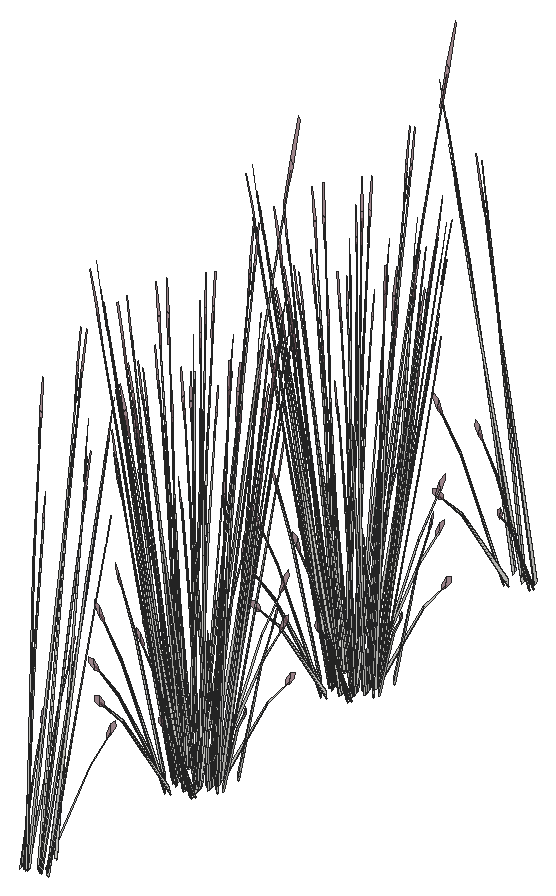
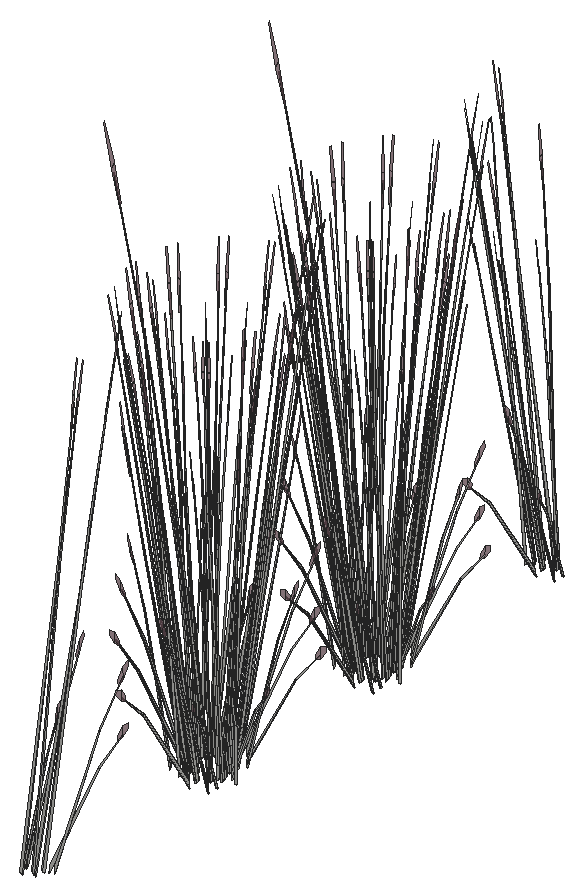
# SketchUp Ruby script. Lengths in inches.
U = 1.inch
M = Sketchup.active_model
def pt(a) = Geom::Point3d.new(a.map { |v| v * U })
def face(e, loops, mat)
  f = e.add_face(loops[0].map { |a| pt(a) })
  loops[1..].each { |l| e.add_face(l.map { |a| pt(a) }).erase! }
  f.material = f.back_material = mat if mat
  f
end
# faces: each face lists its corners as indices into pts; further lists are holes
def faces(e, pts, list, mat = nil) = list.each { |f| face(e, (f[0].is_a?(Array) ? f : [f]).map { |l| l.map { |i| pts[i] } }, mat) }
# xy, xz, yz: faces in a plane at the given z, y or x. An outline is a flat list of corners, or four numbers for a rectangle; further outlines are holes
def ring(l) = l.size == 4 ? [[l[0], l[1]], [l[2], l[1]], [l[2], l[3]], [l[0], l[3]]] : l.each_slice(2).to_a
def flat(e, list, mat, &to3) = list.each { |f| face(e, (f[0].is_a?(Array) ? f : [f]).map { |l| ring(l).map { |u, v| to3.(u, v) } }, mat) }
def xy(e, z, list, mat = nil) = flat(e, list, mat) { |x, y| [x, y, z] }
def xz(e, y, list, mat = nil) = flat(e, list, mat) { |x, z| [x, y, z] }
def yz(e, x, list, mat = nil) = flat(e, list, mat) { |y, z| [x, y, z] }
def lines(e, pts, list) = list.each { |a, b| e.add_line(pt(pts[a]), pt(pts[b])) }
# prism: a flat outline (further loops are holes) pulled along v
def prism(e, loops, v, mat = nil)
  f = face(e, loops, mat); d = Geom::Vector3d.new(v.map { |x| x * U })
  f.pushpull(f.normal.samedirection?(d) ? d.length : -d.length)
end
def box(e, o, s, mat = nil) = prism(e, [[o, [o[0] + s[0], o[1], o[2]], [o[0] + s[0], o[1] + s[1], o[2]], [o[0], o[1] + s[1], o[2]]]], [0, 0, s[2]], mat)
def at(x, y, z, deg = 0) = Geom::Transformation.translation(pt([x, y, z])) * Geom::Transformation.rotation(ORIGIN, Z_AXIS, deg.degrees)
def axes(o, x, y, z) = Geom::Transformation.new([*x, 0, *y, 0, *z, 0, *pt(o).to_a, 1])
def part(name) = M.definitions.add(name)
# library, detail: a bought-in or finely detailed component or shape, given as its bounding box
def library(name, o, s) = part(name).tap { |d| box(d.entities, o, s) }
def detail(e, o, s) = box(e.add_group.entities, o, s)
def put(e, d, t, mat = nil) = e.add_instance(d, t).tap { |i| i.material = mat if mat }
def group(e, t, mat = nil) = e.add_group.tap { |g| g.transformation = t; g.material = mat if mat }.entities
root = M.entities
M.materials.add("LightPink_Translucent").color = [144, 107, 117]
M.materials["LightPink_Translucent"].alpha = 0.75
c1 = part("blade")
p = [[2.15,0.21,22],[0,0.17,0],[0.09,0.45,0],[2.18,0.31,22],[2.29,0.31,22],[0.38,0.45,0],
  [2.48,0.24,33],[2.49,0.24,33],[2.48,0.22,33]]
faces(c1.entities,p,[[0,1,2,3],[4,5,2,3],[6,3,4,7],[8,0,3,6]])
c2 = part("seeds")
p = [[0.3,-0.1,1.38],[-0.01,-0.03,1.59],[-0.01,-0.03,0.03],[0.14,-0.07,-0.07],[0.29,-0.03,3],[0.15,0.01,3.11]]
faces(c2.entities,p,[[0,1,2,3],[1,0,4,5]],"LightPink_Translucent")
c3 = part("blade with seeds")
put(c3.entities,c1,at(0,0,0))
put(c3.entities,c2,axes([2.4,0.25,30.99],[1.5799,-0.05474,1.17369],[-0.12525,1.92788,0.29478],[-0.07173,-0.02425,1.56792]))
put(root,c3,axes([400.88,582.56,4.73],[-0.29004,-0.02173,0.0643],[0.00795,-0.32812,0.50621],[-0.03035,0.12569,0.77189]))
put(root,c3,axes([400.98,582.59,4.73],[-0.25132,-0.3182,0.48003],[0.2669,-0.27442,0.3958],[-0.04636,0.14929,0.9933]))
put(root,c3,axes([401.77,582.75,5.05],[0.1064,-0.35863,0.35414],[0.31043,0.1046,-0.4572],[0.02846,0.14439,0.87481]))
put(root,c3,axes([402.56,583.03,4.73],[-0.16041,0.29625,0.0643],[-0.22843,-0.17248,0.50621],[0.07385,0.09498,0.77189]))
put(root,c3,axes([402.1875,584.03,5.65],[0.2439,-0.26754,-0.06488],[0.22348,0.29302,-0.29416],[0.01573,0.08303,0.97024]))
put(root,c3,axes([402.63,582.94,4.73],[-0.35104,0.10702,0.48003],[-0.06092,-0.41983,0.3958],[0.08256,0.12373,0.9933]))
put(root,c3,axes([401.67,583.07,4.73],[-0.26007,0.1585,0.0643],[-0.12729,-0.28902,0.50621],[0.02512,0.1274,0.77189]))
put(root,c3,axes([400.15,582.62,4.72],[-0.00877,0.09229,1.74944],[0.24897,0.32105,-0.27667],[-0.06518,0.15182,0.14031]))
put(root,c3,axes([400.95,582.41,5.4],[0.3879,0.02311,-0.13498],[-0.0106,0.43749,-0.74919],[-0.02694,0.1685,1.13838]))
put(root,c3,axes([401.67,582.9,5.03],[0.34538,-0.21713,-0.1216],[0.16972,0.38536,-0.67495],[0.04557,0.16239,1.02557]))
put(root,c3,axes([401.77,583.04,5.0625],[-0.34777,-0.12192,0.53283],[0.11892,-0.40083,0.43934],[0.0209,0.15763,1.10256]))
put(root,c3,axes([400.125,583.5625,4.71],[0.04004,-0.02816,1.77383],[0.33095,0.18728,-0.16761],[-0.00778,0.15594,0.31391]))
put(root,c3,axes([401.58,583.76,4.72],[0.04474,0.0751,1.74944],[0.36104,0.0295,-0.27667],[0.03631,0.16562,0.14031]))
put(root,c3,axes([401.89,597.5625,4.72],[-0.05398,-0.06539,1.74944],[-0.36026,0.04145,-0.27667],[-0.0575,-0.15639,0.14031]))
put(root,c3,axes([403.51,598.36,4.72],[-0.00341,-0.09282,1.74944],[-0.28775,-0.26825,-0.27667],[0.04449,-0.16261,0.14031]))
put(root,c3,axes([403.43,598.03,4.71],[-0.03584,0.03562,1.77383],[-0.35118,-0.12018,-0.16761],[-0.01271,-0.15545,0.31391]))
put(root,c3,axes([401.52,597.35,4.71],[-0.00658,0.0559,1.77383],[-0.32474,0.20287,-0.16761],[-0.09556,-0.1037,0.31391]))
put(root,c3,axes([401.45,598.34,5.09],[0.39316,-0.11987,0.53763],[0.06823,0.47021,0.4433],[-0.09247,-0.13858,1.11249]))
put(root,c3,axes([402.34,598.43,4.73],[0.34777,0.12192,0.48003],[-0.11892,0.40083,0.3958],[-0.0209,-0.15763,0.9933]))
put(root,c3,axes([402.4375,598.57,5.03],[-0.34538,0.21713,-0.1216],[-0.16972,-0.38536,-0.67495],[-0.04557,-0.16239,1.02557]))
put(root,c3,axes([403.15,599.06,5.03],[-0.3879,-0.02311,-0.1216],[0.0106,-0.43749,-0.67495],[0.02694,-0.1685,1.02557]))
put(root,c3,axes([402.43,598.4,4.73],[0.26007,-0.1585,0.0643],[0.12729,0.28902,0.50621],[-0.02512,-0.1274,0.77189]))
put(root,c3,axes([401.54,598.44,4.73],[0.16041,-0.29625,0.0643],[0.22843,0.17248,0.50621],[-0.07385,-0.09498,0.77189]))
put(root,c3,axes([402.33,598.72,5.05],[-0.1064,0.35863,0.35414],[-0.31043,-0.1046,-0.4572],[-0.02846,-0.14439,0.87481]))
put(root,c3,axes([403.125,598.875,4.73],[0.25132,0.3182,0.48003],[-0.2669,0.27442,0.3958],[0.04636,-0.14929,0.9933]))
put(root,c3,axes([401.61,598.41,5.43],[-0.23555,0.44708,-0.13619],[-0.34112,-0.25757,-0.75594],[-0.11858,-0.12631,1.14864]))
put(root,c3,axes([403.22,598.9,4.73],[0.29004,0.02173,0.0643],[-0.00795,0.32812,0.50621],[0.03035,-0.12569,0.77189]))
put(root,c3,axes([403,599.125,5.05],[-0.23881,0.24554,0.35414],[-0.22606,-0.28036,-0.4572],[0.0344,-0.14245,0.87481]))
put(root,c3,axes([400.71,598.28,4.72],[-0.07594,-0.00329,1.74944],[-0.24177,0.32918,-0.27667],[-0.129,-0.06726,0.14031]))
put(root,c3,axes([403.58,599.92,5.03],[-0.32648,-0.25715,-0.1216],[0.18809,-0.3724,-0.67495],[0.09224,-0.12945,1.02557]))
put(root,c3,axes([401.59,598.78,5.05],[0.05451,0.37564,0.35414],[-0.31161,0.09919,-0.4572],[-0.0837,-0.10765,0.87481]))
put(root,c3,axes([400.65,599.03,5.09],[0.29147,-0.34417,0.53763],[0.25138,0.3655,0.4433],[-0.13675,-0.06349,1.11249]))
put(root,c3,axes([404.38,599.81,4.71],[-0.0461,-0.00354,1.77383],[-0.19143,-0.37951,-0.16761],[0.07688,-0.12478,0.31391]))
put(root,c3,axes([400.78,599.03,4.73],[0.01777,-0.35463,0.0643],[0.26836,0.00972,0.50621],[-0.1028,-0.03711,0.77189]))
put(root,c3,axes([403.42,599.89,5.05],[-0.30722,0.06665,0.35414],[-0.08112,-0.381,-0.4572],[0.08804,-0.10234,0.87481]))
put(root,c3,axes([403.7,599.83,4.73],[0.2423,0.19613,0.0643],[-0.14107,0.2793,0.50621],[0.07768,-0.0903,0.77189]))
put(root,c3,axes([403.63,599.74,4.73],[0.08753,0.42921,0.48003],[-0.34336,0.07449,0.3958],[0.1012,-0.10094,0.9933]))
put(root,c3,axes([404.55,600.26,4.72],[0.04898,-0.07104,1.74944],[-0.06269,-0.43574,-0.27667],[0.12289,-0.08262,0.14031]))
put(root,c3,axes([400.42,598.5625,4.71],[0.02617,0.04654,1.77383],[-0.12614,0.41836,-0.16761],[-0.12775,0.00303,0.31391]))
put(root,c3,axes([400.97,599.29,5.05],[0.20082,0.29199,0.35414],[-0.2293,0.2764,-0.4572],[-0.1165,-0.04206,0.87481]))
put(root,c3,axes([400.91,599.1,5.03],[-0.0189,0.47427,-0.1216],[-0.35781,-0.01296,-0.67495],[-0.13781,-0.03295,1.02557]))
put(root,c3,axes([403.59,600.92,5.03],[-0.17758,-0.42229,-0.1216],[0.31518,-0.20752,-0.67495],[0.13282,-0.05572,1.02557]))
put(root,c3,axes([403.47,600.8,5.05],[-0.29332,-0.1301,0.35414],[0.08555,-0.37955,-0.4572],[0.11809,-0.0348,0.87481]))
put(root,c3,axes([400.4,600.1,4.73],[0.09971,-0.42522,0.48003],[0.32782,0.1454,0.3958],[-0.12892,0.02555,0.9933]))
put(root,c3,axes([400.37,599.99,4.73],[-0.12963,-0.31798,0.0643],[0.23638,-0.15564,0.50621],[-0.1042,0.03071,0.77189]))
put(root,c3,axes([403.73,600.92,4.73],[0.12963,0.31798,0.0643],[-0.23638,0.15564,0.50621],[0.1042,-0.03071,0.77189]))
put(root,c3,axes([403.71,600.8,4.73],[-0.09971,0.42522,0.48003],[-0.32782,-0.1454,0.3958],[0.12892,-0.02555,0.9933]))
put(root,c3,axes([400.64,600.11,5.05],[0.29332,0.1301,0.35414],[-0.08555,0.37955,-0.4572],[-0.11809,0.0348,0.87481]))
put(root,c3,axes([404.3,602.18,4.71],[-0.03191,-0.04083,1.77383],[0.06981,-0.43764,-0.16761],[0.12571,-0.02796,0.31391]))
put(root,c3,axes([400.14,600.4,4.72],[-0.05763,0.06055,1.74944],[0.0049,0.44239,-0.27667],[-0.13211,0.05753,0.14031]))
put(root,c3,axes([400.51,599.98,5.03],[0.17758,0.42229,-0.1216],[-0.31518,0.20752,-0.67495],[-0.13282,0.05572,1.02557]))
put(root,c3,axes([403.19,601.8,5.03],[0.0189,-0.47427,-0.1216],[0.35781,0.01296,-0.67495],[0.13781,0.03295,1.02557]))
put(root,c3,axes([403.14,601.62,5.05],[-0.20082,-0.29199,0.35414],[0.2293,-0.2764,-0.4572],[0.1165,0.04206,0.87481]))
put(root,c3,axes([403.5,601.52,4.72],[0.07571,-0.00789,1.74944],[0.20767,-0.36231,-0.27667],[0.13467,0.04783,0.14031]))
put(root,c3,axes([400.47,601.16,4.73],[-0.08753,-0.42921,0.48003],[0.34336,-0.07449,0.3958],[-0.1012,0.10094,0.9933]))
put(root,c3,axes([400.41,601.08,4.73],[-0.2423,-0.19613,0.0643],[0.14107,-0.2793,0.50621],[-0.07768,0.0903,0.77189]))
put(root,c3,axes([400.6875,601.02,5.05],[0.30722,-0.06665,0.35414],[0.08112,0.381,-0.4572],[-0.08804,0.10234,0.87481]))
put(root,c3,axes([399.5,600.85,4.71],[0.04504,0.01251,1.77383],[0.13934,0.41205,-0.16761],[-0.0922,0.10815,0.31391]))
put(root,c3,axes([403.32,601.88,4.73],[-0.01777,0.35463,0.0643],[-0.26836,-0.00972,0.50621],[0.1028,0.03711,0.77189]))
put(root,c3,axes([403.34,601.77,4.73],[-0.26024,0.30729,0.48003],[-0.22444,-0.32634,0.3958],[0.1221,0.05668,0.9933]))
put(root,c3,axes([399.99,602.1,5.65],[0.31145,0.12449,-0.06488],[-0.0958,0.38314,-0.29416],[-0.05094,0.05817,0.97024]))
put(root,c3,axes([402.52,602.125,5.05],[-0.05451,-0.37564,0.35414],[0.31161,-0.09919,-0.4572],[0.0837,0.10765,0.87481]))
put(root,c3,axes([402.72,599.96,4.47],[-0.30498,-0.24231,1.38283],[0.32203,-0.37727,0.59665],[0.0984,0.22736,1.33663]))
put(root,c3,axes([400.53,600.99,5.03],[0.32648,0.25715,-0.1216],[-0.18809,0.3724,-0.67495],[-0.09224,0.12945,1.02557]))
put(root,c3,axes([402.49,602.32,5.03],[0.21031,-0.39918,-0.1216],[0.30457,0.22997,-0.67495],[0.10587,0.11278,1.02557]))
put(root,c3,axes([401.1,601.78,5.05],[0.23881,-0.24554,0.35414],[0.22606,0.28036,-0.4572],[-0.0344,0.14245,0.87481]))
put(root,c3,axes([402.21,602.65,4.71],[0.00104,-0.05646,1.77383],[0.30246,-0.2491,-0.16761],[0.10506,0.08891,0.31391]))
put(root,c3,axes([400.88,602,4.73],[-0.29004,-0.02173,0.0643],[0.00795,-0.32812,0.50621],[-0.03035,0.12569,0.77189]))
put(root,c3,axes([400.98,602.03,4.73],[-0.25132,-0.3182,0.48003],[0.2669,-0.27442,0.3958],[-0.04636,0.14929,0.9933]))
put(root,c3,axes([401.77,602.18,5.05],[0.1064,-0.35863,0.35414],[0.31043,0.1046,-0.4572],[0.02846,0.14439,0.87481]))
put(root,c3,axes([402.56,602.46,4.73],[-0.16041,0.29625,0.0643],[-0.22843,-0.17248,0.50621],[0.07385,0.09498,0.77189]))
put(root,c3,axes([402.1875,603.46,5.65],[0.2439,-0.26754,-0.06488],[0.22348,0.29302,-0.29416],[0.01573,0.08303,0.97024]))
put(root,c3,axes([402.63,602.38,4.73],[-0.35104,0.10702,0.48003],[-0.06092,-0.41983,0.3958],[0.08256,0.12373,0.9933]))
put(root,c3,axes([401.67,602.51,4.73],[-0.26007,0.1585,0.0643],[-0.12729,-0.28902,0.50621],[0.02512,0.1274,0.77189]))
put(root,c3,axes([400.15,602.05,4.72],[-0.00877,0.09229,1.74944],[0.24897,0.32105,-0.27667],[-0.06518,0.15182,0.14031]))
put(root,c3,axes([400.95,601.85,5.4],[0.3879,0.02311,-0.13498],[-0.0106,0.43749,-0.74919],[-0.02694,0.1685,1.13838]))
put(root,c3,axes([401.67,602.33,5.03],[0.34538,-0.21713,-0.1216],[0.16972,0.38536,-0.67495],[0.04557,0.16239,1.02557]))
put(root,c3,axes([401.77,602.48,5.0625],[-0.34777,-0.12192,0.53283],[0.11892,-0.40083,0.43934],[0.0209,0.15763,1.10256]))
put(root,c3,axes([400.125,603,4.71],[0.04004,-0.02816,1.77383],[0.33095,0.18728,-0.16761],[-0.00778,0.15594,0.31391]))
put(root,c3,axes([401.58,603.2,4.72],[0.04474,0.0751,1.74944],[0.36104,0.0295,-0.27667],[0.03631,0.16562,0.14031]))
put(root,c3,axes([401.89,615.15,4.72],[-0.05398,-0.06539,1.74944],[-0.36026,0.04145,-0.27667],[-0.0575,-0.15639,0.14031]))
put(root,c3,axes([403.51,615.95,4.72],[-0.00341,-0.09282,1.74944],[-0.28775,-0.26825,-0.27667],[0.04449,-0.16261,0.14031]))
put(root,c3,axes([403.43,615.61,4.71],[-0.03584,0.03562,1.77383],[-0.35118,-0.12018,-0.16761],[-0.01271,-0.15545,0.31391]))
put(root,c3,axes([401.52,614.93,4.71],[-0.00658,0.0559,1.77383],[-0.32474,0.20287,-0.16761],[-0.09556,-0.1037,0.31391]))
put(root,c3,axes([401.45,615.92,5.09],[0.39316,-0.11987,0.53763],[0.06823,0.47021,0.4433],[-0.09247,-0.13858,1.11249]))
put(root,c3,axes([402.34,616.01,4.73],[0.34777,0.12192,0.48003],[-0.11892,0.40083,0.3958],[-0.0209,-0.15763,0.9933]))
put(root,c3,axes([402.4375,616.15,5.03],[-0.34538,0.21713,-0.1216],[-0.16972,-0.38536,-0.67495],[-0.04557,-0.16239,1.02557]))
put(root,c3,axes([403.15,616.64,5.03],[-0.3879,-0.02311,-0.1216],[0.0106,-0.43749,-0.67495],[0.02694,-0.1685,1.02557]))
put(root,c3,axes([402.43,615.98,4.73],[0.26007,-0.1585,0.0643],[0.12729,0.28902,0.50621],[-0.02512,-0.1274,0.77189]))
put(root,c3,axes([401.54,616.03,4.73],[0.16041,-0.29625,0.0643],[0.22843,0.17248,0.50621],[-0.07385,-0.09498,0.77189]))
put(root,c3,axes([402.33,616.31,5.05],[-0.1064,0.35863,0.35414],[-0.31043,-0.1046,-0.4572],[-0.02846,-0.14439,0.87481]))
put(root,c3,axes([403.125,616.46,4.73],[0.25132,0.3182,0.48003],[-0.2669,0.27442,0.3958],[0.04636,-0.14929,0.9933]))
put(root,c3,axes([401.61,615.99,5.43],[-0.23555,0.44708,-0.13619],[-0.34112,-0.25757,-0.75594],[-0.11858,-0.12631,1.14864]))
put(root,c3,axes([403.22,616.49,4.73],[0.29004,0.02173,0.0643],[-0.00795,0.32812,0.50621],[0.03035,-0.12569,0.77189]))
put(root,c3,axes([403,616.71,5.05],[-0.23881,0.24554,0.35414],[-0.22606,-0.28036,-0.4572],[0.0344,-0.14245,0.87481]))
put(root,c3,axes([400.71,615.87,4.72],[-0.07594,-0.00329,1.74944],[-0.24177,0.32918,-0.27667],[-0.129,-0.06726,0.14031]))
put(root,c3,axes([403.58,617.5,5.03],[-0.32648,-0.25715,-0.1216],[0.18809,-0.3724,-0.67495],[0.09224,-0.12945,1.02557]))
put(root,c3,axes([401.59,616.37,5.05],[0.05451,0.37564,0.35414],[-0.31161,0.09919,-0.4572],[-0.0837,-0.10765,0.87481]))
put(root,c3,axes([400.65,616.61,5.09],[0.29147,-0.34417,0.53763],[0.25138,0.3655,0.4433],[-0.13675,-0.06349,1.11249]))
put(root,c3,axes([404.38,617.39,4.71],[-0.0461,-0.00354,1.77383],[-0.19143,-0.37951,-0.16761],[0.07688,-0.12478,0.31391]))
put(root,c3,axes([400.78,616.61,4.73],[0.01777,-0.35463,0.0643],[0.26836,0.00972,0.50621],[-0.1028,-0.03711,0.77189]))
put(root,c3,axes([403.42,617.47,5.05],[-0.30722,0.06665,0.35414],[-0.08112,-0.381,-0.4572],[0.08804,-0.10234,0.87481]))
put(root,c3,axes([403.7,617.41,4.73],[0.2423,0.19613,0.0643],[-0.14107,0.2793,0.50621],[0.07768,-0.0903,0.77189]))
put(root,c3,axes([403.63,617.33,4.73],[0.08753,0.42921,0.48003],[-0.34336,0.07449,0.3958],[0.1012,-0.10094,0.9933]))
put(root,c3,axes([404.55,617.85,4.72],[0.04898,-0.07104,1.74944],[-0.06269,-0.43574,-0.27667],[0.12289,-0.08262,0.14031]))
put(root,c3,axes([400.42,616.14,4.71],[0.02617,0.04654,1.77383],[-0.12614,0.41836,-0.16761],[-0.12775,0.00303,0.31391]))
put(root,c3,axes([400.97,616.87,5.05],[0.20082,0.29199,0.35414],[-0.2293,0.2764,-0.4572],[-0.1165,-0.04206,0.87481]))
put(root,c3,axes([400.91,616.6875,5.03],[-0.0189,0.47427,-0.1216],[-0.35781,-0.01296,-0.67495],[-0.13781,-0.03295,1.02557]))
put(root,c3,axes([403.59,618.51,5.03],[-0.17758,-0.42229,-0.1216],[0.31518,-0.20752,-0.67495],[0.13282,-0.05572,1.02557]))
put(root,c3,axes([403.47,618.38,5.05],[-0.29332,-0.1301,0.35414],[0.08555,-0.37955,-0.4572],[0.11809,-0.0348,0.87481]))
put(root,c3,axes([400.4,617.6875,4.73],[0.09971,-0.42522,0.48003],[0.32782,0.1454,0.3958],[-0.12892,0.02555,0.9933]))
put(root,c3,axes([400.37,617.57,4.73],[-0.12963,-0.31798,0.0643],[0.23638,-0.15564,0.50621],[-0.1042,0.03071,0.77189]))
put(root,c3,axes([403.73,618.5,4.73],[0.12963,0.31798,0.0643],[-0.23638,0.15564,0.50621],[0.1042,-0.03071,0.77189]))
put(root,c3,axes([403.71,618.39,4.73],[-0.09971,0.42522,0.48003],[-0.32782,-0.1454,0.3958],[0.12892,-0.02555,0.9933]))
put(root,c3,axes([400.64,617.69,5.05],[0.29332,0.1301,0.35414],[-0.08555,0.37955,-0.4572],[-0.11809,0.0348,0.87481]))
put(root,c3,axes([404.3,619.76,4.71],[-0.03191,-0.04083,1.77383],[0.06981,-0.43764,-0.16761],[0.12571,-0.02796,0.31391]))
put(root,c3,axes([400.14,617.99,4.72],[-0.05763,0.06055,1.74944],[0.0049,0.44239,-0.27667],[-0.13211,0.05753,0.14031]))
put(root,c3,axes([400.51,617.5625,5.03],[0.17758,0.42229,-0.1216],[-0.31518,0.20752,-0.67495],[-0.13282,0.05572,1.02557]))
put(root,c3,axes([403.19,619.38,5.03],[0.0189,-0.47427,-0.1216],[0.35781,0.01296,-0.67495],[0.13781,0.03295,1.02557]))
put(root,c3,axes([403.14,619.2,5.05],[-0.20082,-0.29199,0.35414],[0.2293,-0.2764,-0.4572],[0.1165,0.04206,0.87481]))
put(root,c3,axes([403.5,619.1,4.72],[0.07571,-0.00789,1.74944],[0.20767,-0.36231,-0.27667],[0.13467,0.04783,0.14031]))
put(root,c3,axes([400.47,618.75,4.73],[-0.08753,-0.42921,0.48003],[0.34336,-0.07449,0.3958],[-0.1012,0.10094,0.9933]))
put(root,c3,axes([400.41,618.66,4.73],[-0.2423,-0.19613,0.0643],[0.14107,-0.2793,0.50621],[-0.07768,0.0903,0.77189]))
put(root,c3,axes([400.6875,618.6,5.05],[0.30722,-0.06665,0.35414],[0.08112,0.381,-0.4572],[-0.08804,0.10234,0.87481]))
put(root,c3,axes([399.5,618.43,4.71],[0.04504,0.01251,1.77383],[0.13934,0.41205,-0.16761],[-0.0922,0.10815,0.31391]))
put(root,c3,axes([403.32,619.46,4.73],[-0.01777,0.35463,0.0643],[-0.26836,-0.00972,0.50621],[0.1028,0.03711,0.77189]))
put(root,c3,axes([403.34,619.35,4.73],[-0.26024,0.30729,0.48003],[-0.22444,-0.32634,0.3958],[0.1221,0.05668,0.9933]))
put(root,c3,axes([399.99,619.68,5.65],[0.31145,0.12449,-0.06488],[-0.0958,0.38314,-0.29416],[-0.05094,0.05817,0.97024]))
put(root,c3,axes([402.52,619.71,5.05],[-0.05451,-0.37564,0.35414],[0.31161,-0.09919,-0.4572],[0.0837,0.10765,0.87481]))
put(root,c3,axes([402.72,617.55,4.47],[-0.30498,-0.24231,1.38283],[0.32203,-0.37727,0.59665],[0.0984,0.22736,1.33663]))
put(root,c3,axes([400.53,618.57,5.03],[0.32648,0.25715,-0.1216],[-0.18809,0.3724,-0.67495],[-0.09224,0.12945,1.02557]))
put(root,c3,axes([402.49,619.9,5.03],[0.21031,-0.39918,-0.1216],[0.30457,0.22997,-0.67495],[0.10587,0.11278,1.02557]))
put(root,c3,axes([401.1,619.36,5.05],[0.23881,-0.24554,0.35414],[0.22606,0.28036,-0.4572],[-0.0344,0.14245,0.87481]))
put(root,c3,axes([402.21,620.23,4.71],[0.00104,-0.05646,1.77383],[0.30246,-0.2491,-0.16761],[0.10506,0.08891,0.31391]))
put(root,c3,axes([400.88,619.58,4.73],[-0.29004,-0.02173,0.0643],[0.00795,-0.32812,0.50621],[-0.03035,0.12569,0.77189]))
put(root,c3,axes([400.98,619.61,4.73],[-0.25132,-0.3182,0.48003],[0.2669,-0.27442,0.3958],[-0.04636,0.14929,0.9933]))
put(root,c3,axes([401.77,619.77,5.05],[0.1064,-0.35863,0.35414],[0.31043,0.1046,-0.4572],[0.02846,0.14439,0.87481]))
put(root,c3,axes([402.56,620.05,4.73],[-0.16041,0.29625,0.0643],[-0.22843,-0.17248,0.50621],[0.07385,0.09498,0.77189]))
put(root,c3,axes([402.1875,621.05,5.65],[0.2439,-0.26754,-0.06488],[0.22348,0.29302,-0.29416],[0.01573,0.08303,0.97024]))
put(root,c3,axes([402.63,619.96,4.73],[-0.35104,0.10702,0.48003],[-0.06092,-0.41983,0.3958],[0.08256,0.12373,0.9933]))
put(root,c3,axes([401.67,620.09,4.73],[-0.26007,0.1585,0.0643],[-0.12729,-0.28902,0.50621],[0.02512,0.1274,0.77189]))
put(root,c3,axes([400.15,619.64,4.72],[-0.00877,0.09229,1.74944],[0.24897,0.32105,-0.27667],[-0.06518,0.15182,0.14031]))
put(root,c3,axes([400.95,619.43,5.4],[0.3879,0.02311,-0.13498],[-0.0106,0.43749,-0.74919],[-0.02694,0.1685,1.13838]))
put(root,c3,axes([401.67,619.92,5.03],[0.34538,-0.21713,-0.1216],[0.16972,0.38536,-0.67495],[0.04557,0.16239,1.02557]))
put(root,c3,axes([401.77,620.06,5.0625],[-0.34777,-0.12192,0.53283],[0.11892,-0.40083,0.43934],[0.0209,0.15763,1.10256]))
put(root,c3,axes([400.125,620.58,4.71],[0.04004,-0.02816,1.77383],[0.33095,0.18728,-0.16761],[-0.00778,0.15594,0.31391]))
put(root,c3,axes([401.58,620.78,4.72],[0.04474,0.0751,1.74944],[0.36104,0.0295,-0.27667],[0.03631,0.16562,0.14031]))
put(root,c3,axes([401.89,635.68,4.72],[-0.05398,-0.06539,1.74944],[-0.36026,0.04145,-0.27667],[-0.0575,-0.15639,0.14031]))
put(root,c3,axes([403.51,636.48,4.72],[-0.00341,-0.09282,1.74944],[-0.28775,-0.26825,-0.27667],[0.04449,-0.16261,0.14031]))
put(root,c3,axes([403.43,636.15,4.71],[-0.03584,0.03562,1.77383],[-0.35118,-0.12018,-0.16761],[-0.01271,-0.15545,0.31391]))
put(root,c3,axes([401.52,635.47,4.71],[-0.00658,0.0559,1.77383],[-0.32474,0.20287,-0.16761],[-0.09556,-0.1037,0.31391]))
put(root,c3,axes([401.45,636.46,5.09],[0.39316,-0.11987,0.53763],[0.06823,0.47021,0.4433],[-0.09247,-0.13858,1.11249]))
put(root,c3,axes([402.34,636.55,4.73],[0.34777,0.12192,0.48003],[-0.11892,0.40083,0.3958],[-0.0209,-0.15763,0.9933]))
put(root,c3,axes([402.4375,636.69,5.03],[-0.34538,0.21713,-0.1216],[-0.16972,-0.38536,-0.67495],[-0.04557,-0.16239,1.02557]))
put(root,c3,axes([403.15,637.18,5.03],[-0.3879,-0.02311,-0.1216],[0.0106,-0.43749,-0.67495],[0.02694,-0.1685,1.02557]))
